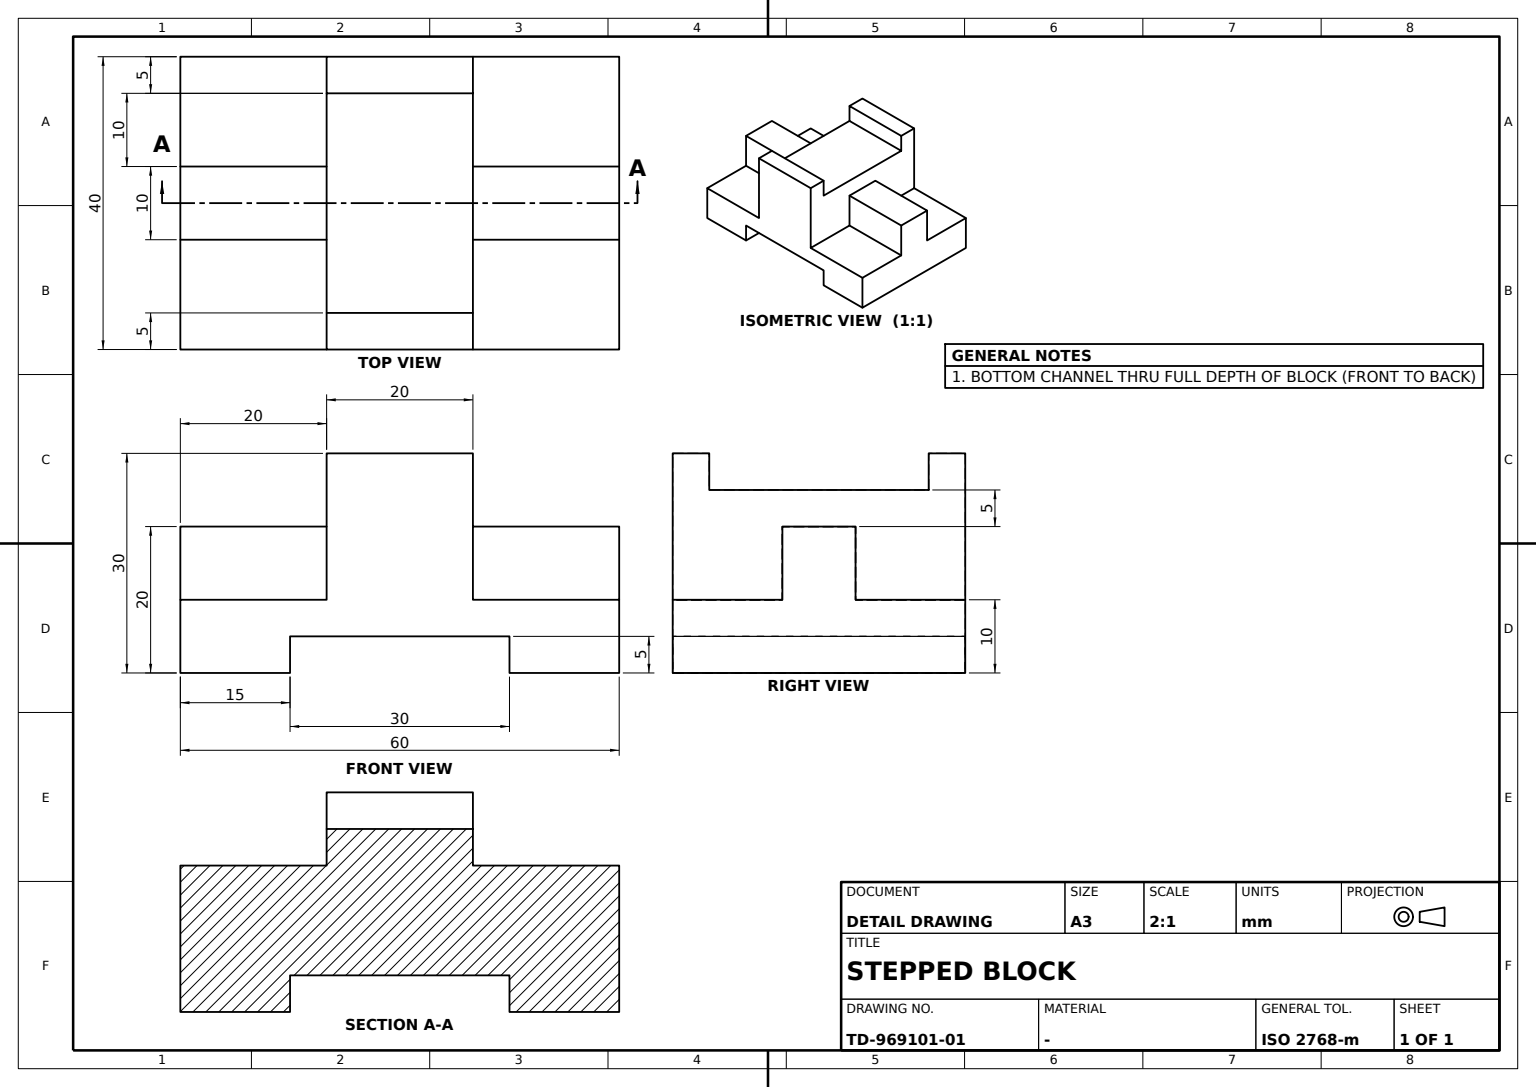
ISO-10303-21;
HEADER;
FILE_DESCRIPTION((''),'2;1');
FILE_NAME('','',(''),(''),'','','');
FILE_SCHEMA(('AUTOMOTIVE_DESIGN'));
ENDSEC;
DATA;
#1=APPLICATION_CONTEXT('');
#2=PRODUCT_CONTEXT('',#1,'mechanical');
#3=PRODUCT('','','',(#2));
#4=PRODUCT_DEFINITION_FORMATION('','',#3);
#5=PRODUCT_DEFINITION_CONTEXT('',#1,'design');
#6=PRODUCT_DEFINITION('','',#4,#5);
#7=PRODUCT_DEFINITION_SHAPE('','',#6);
#8=(LENGTH_UNIT()NAMED_UNIT(*)SI_UNIT(.MILLI.,.METRE.));
#9=(NAMED_UNIT(*)PLANE_ANGLE_UNIT()SI_UNIT($,.RADIAN.));
#10=(NAMED_UNIT(*)SI_UNIT($,.STERADIAN.)SOLID_ANGLE_UNIT());
#11=UNCERTAINTY_MEASURE_WITH_UNIT(LENGTH_MEASURE(0.005),#8,'distance_accuracy_value','');
#12=(GEOMETRIC_REPRESENTATION_CONTEXT(3)GLOBAL_UNCERTAINTY_ASSIGNED_CONTEXT((#11))GLOBAL_UNIT_ASSIGNED_CONTEXT((#8,#9,#10))REPRESENTATION_CONTEXT('',''));
#13=CARTESIAN_POINT('',(-10.,-5.,25.));
#14=VERTEX_POINT('',#13);
#15=CARTESIAN_POINT('',(-10.,-35.,25.));
#16=VERTEX_POINT('',#15);
#17=DIRECTION('',(0.,-1.,0.));
#18=VECTOR('',#17,1000.);
#19=LINE('',#13,#18);
#20=EDGE_CURVE('',#14,#16,#19,.T.);
#21=ORIENTED_EDGE('',*,*,#20,.T.);
#22=CARTESIAN_POINT('',(10.,-35.,25.));
#23=VERTEX_POINT('',#22);
#24=CARTESIAN_POINT('',(0.,-35.,25.));
#25=DIRECTION('',(-1.,0.,0.));
#26=VECTOR('',#25,1000.);
#27=LINE('',#24,#26);
#28=EDGE_CURVE('',#23,#16,#27,.T.);
#29=ORIENTED_EDGE('',*,*,#28,.F.);
#30=CARTESIAN_POINT('',(10.,-5.,25.));
#31=VERTEX_POINT('',#30);
#32=CARTESIAN_POINT('',(10.,0.,25.));
#33=LINE('',#32,#18);
#34=EDGE_CURVE('',#31,#23,#33,.T.);
#35=ORIENTED_EDGE('',*,*,#34,.F.);
#36=CARTESIAN_POINT('',(0.,-5.,25.));
#37=LINE('',#36,#26);
#38=EDGE_CURVE('',#31,#14,#37,.T.);
#39=ORIENTED_EDGE('',*,*,#38,.T.);
#40=EDGE_LOOP('',(#21,#29,#35,#39));
#41=FACE_BOUND('',#40,.T.);
#42=DIRECTION('',(0.,0.,-1.));
#43=AXIS2_PLACEMENT_3D('',#36,#42,#17);
#44=PLANE('',#43);
#45=ADVANCED_FACE('',(#41),#44,.F.);
#46=CARTESIAN_POINT('',(-10.,-25.,10.));
#47=VERTEX_POINT('',#46);
#48=CARTESIAN_POINT('',(-10.,-40.,10.));
#49=VERTEX_POINT('',#48);
#50=CARTESIAN_POINT('',(-10.,0.,10.));
#51=LINE('',#50,#18);
#52=EDGE_CURVE('',#47,#49,#51,.T.);
#53=ORIENTED_EDGE('',*,*,#52,.F.);
#54=CARTESIAN_POINT('',(-30.,-25.,10.));
#55=VERTEX_POINT('',#54);
#56=CARTESIAN_POINT('',(0.,-25.,10.));
#57=DIRECTION('',(1.,0.,0.));
#58=VECTOR('',#57,1000.);
#59=LINE('',#56,#58);
#60=EDGE_CURVE('',#55,#47,#59,.T.);
#61=ORIENTED_EDGE('',*,*,#60,.F.);
#62=CARTESIAN_POINT('',(-30.,-40.,10.));
#63=VERTEX_POINT('',#62);
#64=CARTESIAN_POINT('',(-30.,0.,10.));
#65=LINE('',#64,#18);
#66=EDGE_CURVE('',#55,#63,#65,.T.);
#67=ORIENTED_EDGE('',*,*,#66,.T.);
#68=LINE('',#62,#58);
#69=EDGE_CURVE('',#63,#49,#68,.T.);
#70=ORIENTED_EDGE('',*,*,#69,.T.);
#71=EDGE_LOOP('',(#53,#61,#67,#70));
#72=FACE_BOUND('',#71,.T.);
#73=AXIS2_PLACEMENT_3D('',#64,#42,#57);
#74=PLANE('',#73);
#75=ADVANCED_FACE('',(#72),#74,.F.);
#76=CARTESIAN_POINT('',(-10.,-25.,20.));
#77=VERTEX_POINT('',#76);
#78=DIRECTION('',(0.,0.,1.));
#79=VECTOR('',#78,1000.);
#80=LINE('',#76,#79);
#81=EDGE_CURVE('',#47,#77,#80,.T.);
#82=ORIENTED_EDGE('',*,*,#81,.T.);
#83=CARTESIAN_POINT('',(-30.,-25.,20.));
#84=VERTEX_POINT('',#83);
#85=CARTESIAN_POINT('',(0.,-25.,20.));
#86=LINE('',#85,#58);
#87=EDGE_CURVE('',#84,#77,#86,.T.);
#88=ORIENTED_EDGE('',*,*,#87,.F.);
#89=CARTESIAN_POINT('',(-30.,-25.,0.));
#90=VECTOR('',#42,1000.);
#91=LINE('',#89,#90);
#92=EDGE_CURVE('',#84,#55,#91,.T.);
#93=ORIENTED_EDGE('',*,*,#92,.T.);
#94=ORIENTED_EDGE('',*,*,#60,.T.);
#95=EDGE_LOOP('',(#82,#88,#93,#94));
#96=FACE_BOUND('',#95,.T.);
#97=AXIS2_PLACEMENT_3D('',#85,#17,#42);
#98=PLANE('',#97);
#99=ADVANCED_FACE('',(#96),#98,.T.);
#100=CARTESIAN_POINT('',(10.,-35.,30.));
#101=VERTEX_POINT('',#100);
#102=CARTESIAN_POINT('',(10.,-40.,30.));
#103=VERTEX_POINT('',#102);
#104=CARTESIAN_POINT('',(10.,0.,30.));
#105=LINE('',#104,#18);
#106=EDGE_CURVE('',#101,#103,#105,.T.);
#107=ORIENTED_EDGE('',*,*,#106,.T.);
#108=CARTESIAN_POINT('',(10.,-40.,10.));
#109=VERTEX_POINT('',#108);
#110=LINE('',#102,#90);
#111=EDGE_CURVE('',#103,#109,#110,.T.);
#112=ORIENTED_EDGE('',*,*,#111,.T.);
#113=CARTESIAN_POINT('',(10.,-25.,10.));
#114=VERTEX_POINT('',#113);
#115=CARTESIAN_POINT('',(10.,0.,10.));
#116=LINE('',#115,#18);
#117=EDGE_CURVE('',#114,#109,#116,.T.);
#118=ORIENTED_EDGE('',*,*,#117,.F.);
#119=CARTESIAN_POINT('',(10.,-25.,20.));
#120=VERTEX_POINT('',#119);
#121=CARTESIAN_POINT('',(10.,-25.,30.));
#122=LINE('',#121,#79);
#123=EDGE_CURVE('',#114,#120,#122,.T.);
#124=ORIENTED_EDGE('',*,*,#123,.T.);
#125=CARTESIAN_POINT('',(10.,-15.,20.));
#126=VERTEX_POINT('',#125);
#127=DIRECTION('',(0.,1.,0.));
#128=VECTOR('',#127,1000.);
#129=LINE('',#119,#128);
#130=EDGE_CURVE('',#120,#126,#129,.T.);
#131=ORIENTED_EDGE('',*,*,#130,.T.);
#132=CARTESIAN_POINT('',(10.,-15.,10.));
#133=VERTEX_POINT('',#132);
#134=LINE('',#132,#79);
#135=EDGE_CURVE('',#133,#126,#134,.T.);
#136=ORIENTED_EDGE('',*,*,#135,.F.);
#137=VERTEX_POINT('',#115);
#138=EDGE_CURVE('',#137,#133,#116,.T.);
#139=ORIENTED_EDGE('',*,*,#138,.F.);
#140=VERTEX_POINT('',#104);
#141=LINE('',#104,#90);
#142=EDGE_CURVE('',#140,#137,#141,.T.);
#143=ORIENTED_EDGE('',*,*,#142,.F.);
#144=CARTESIAN_POINT('',(10.,-5.,30.));
#145=VERTEX_POINT('',#144);
#146=EDGE_CURVE('',#140,#145,#105,.T.);
#147=ORIENTED_EDGE('',*,*,#146,.T.);
#148=LINE('',#144,#79);
#149=EDGE_CURVE('',#31,#145,#148,.T.);
#150=ORIENTED_EDGE('',*,*,#149,.F.);
#151=ORIENTED_EDGE('',*,*,#34,.T.);
#152=LINE('',#100,#90);
#153=EDGE_CURVE('',#101,#23,#152,.T.);
#154=ORIENTED_EDGE('',*,*,#153,.F.);
#155=EDGE_LOOP('',(#107,#112,#118,#124,#131,#136,#139,#143,#147,#150,#151,#154));
#156=FACE_BOUND('',#155,.T.);
#157=AXIS2_PLACEMENT_3D('',#104,#25,#42);
#158=PLANE('',#157);
#159=ADVANCED_FACE('',(#156),#158,.F.);
#160=CARTESIAN_POINT('',(-30.,-15.,10.));
#161=VERTEX_POINT('',#160);
#162=CARTESIAN_POINT('',(-10.,-15.,10.));
#163=VERTEX_POINT('',#162);
#164=LINE('',#160,#58);
#165=EDGE_CURVE('',#161,#163,#164,.T.);
#166=ORIENTED_EDGE('',*,*,#165,.F.);
#167=CARTESIAN_POINT('',(-30.,-15.,20.));
#168=VERTEX_POINT('',#167);
#169=CARTESIAN_POINT('',(-30.,-15.,0.));
#170=LINE('',#169,#79);
#171=EDGE_CURVE('',#161,#168,#170,.T.);
#172=ORIENTED_EDGE('',*,*,#171,.T.);
#173=CARTESIAN_POINT('',(-10.,-15.,20.));
#174=VERTEX_POINT('',#173);
#175=CARTESIAN_POINT('',(0.,-15.,20.));
#176=LINE('',#175,#58);
#177=EDGE_CURVE('',#168,#174,#176,.T.);
#178=ORIENTED_EDGE('',*,*,#177,.T.);
#179=LINE('',#162,#79);
#180=EDGE_CURVE('',#163,#174,#179,.T.);
#181=ORIENTED_EDGE('',*,*,#180,.F.);
#182=EDGE_LOOP('',(#166,#172,#178,#181));
#183=FACE_BOUND('',#182,.T.);
#184=CARTESIAN_POINT('',(0.,-15.,10.));
#185=AXIS2_PLACEMENT_3D('',#184,#127,#78);
#186=PLANE('',#185);
#187=ADVANCED_FACE('',(#183),#186,.T.);
#188=CARTESIAN_POINT('',(30.,0.,10.));
#189=VERTEX_POINT('',#188);
#190=LINE('',#64,#58);
#191=EDGE_CURVE('',#137,#189,#190,.T.);
#192=ORIENTED_EDGE('',*,*,#191,.F.);
#193=ORIENTED_EDGE('',*,*,#138,.T.);
#194=CARTESIAN_POINT('',(30.,-15.,10.));
#195=VERTEX_POINT('',#194);
#196=EDGE_CURVE('',#133,#195,#164,.T.);
#197=ORIENTED_EDGE('',*,*,#196,.T.);
#198=LINE('',#188,#18);
#199=EDGE_CURVE('',#189,#195,#198,.T.);
#200=ORIENTED_EDGE('',*,*,#199,.F.);
#201=EDGE_LOOP('',(#192,#193,#197,#200));
#202=FACE_BOUND('',#201,.T.);
#203=ADVANCED_FACE('',(#202),#74,.F.);
#204=VERTEX_POINT('',#50);
#205=EDGE_CURVE('',#204,#163,#51,.T.);
#206=ORIENTED_EDGE('',*,*,#205,.T.);
#207=ORIENTED_EDGE('',*,*,#180,.T.);
#208=CARTESIAN_POINT('',(-10.,0.,20.));
#209=LINE('',#208,#128);
#210=EDGE_CURVE('',#77,#174,#209,.T.);
#211=ORIENTED_EDGE('',*,*,#210,.F.);
#212=ORIENTED_EDGE('',*,*,#81,.F.);
#213=ORIENTED_EDGE('',*,*,#52,.T.);
#214=CARTESIAN_POINT('',(-10.,-40.,30.));
#215=VERTEX_POINT('',#214);
#216=LINE('',#48,#79);
#217=EDGE_CURVE('',#49,#215,#216,.T.);
#218=ORIENTED_EDGE('',*,*,#217,.T.);
#219=CARTESIAN_POINT('',(-10.,-35.,30.));
#220=VERTEX_POINT('',#219);
#221=CARTESIAN_POINT('',(-10.,0.,30.));
#222=LINE('',#221,#18);
#223=EDGE_CURVE('',#220,#215,#222,.T.);
#224=ORIENTED_EDGE('',*,*,#223,.F.);
#225=LINE('',#219,#90);
#226=EDGE_CURVE('',#220,#16,#225,.T.);
#227=ORIENTED_EDGE('',*,*,#226,.T.);
#228=ORIENTED_EDGE('',*,*,#20,.F.);
#229=CARTESIAN_POINT('',(-10.,-5.,30.));
#230=VERTEX_POINT('',#229);
#231=LINE('',#13,#79);
#232=EDGE_CURVE('',#14,#230,#231,.T.);
#233=ORIENTED_EDGE('',*,*,#232,.T.);
#234=VERTEX_POINT('',#221);
#235=EDGE_CURVE('',#234,#230,#222,.T.);
#236=ORIENTED_EDGE('',*,*,#235,.F.);
#237=LINE('',#50,#79);
#238=EDGE_CURVE('',#204,#234,#237,.T.);
#239=ORIENTED_EDGE('',*,*,#238,.F.);
#240=EDGE_LOOP('',(#206,#207,#211,#212,#213,#218,#224,#227,#228,#233,#236,#239));
#241=FACE_BOUND('',#240,.T.);
#242=AXIS2_PLACEMENT_3D('',#50,#57,#78);
#243=PLANE('',#242);
#244=ADVANCED_FACE('',(#241),#243,.F.);
#245=CARTESIAN_POINT('',(30.,-25.,20.));
#246=VERTEX_POINT('',#245);
#247=CARTESIAN_POINT('',(30.,-25.,10.));
#248=VERTEX_POINT('',#247);
#249=LINE('',#245,#90);
#250=EDGE_CURVE('',#246,#248,#249,.T.);
#251=ORIENTED_EDGE('',*,*,#250,.F.);
#252=EDGE_CURVE('',#120,#246,#86,.T.);
#253=ORIENTED_EDGE('',*,*,#252,.F.);
#254=ORIENTED_EDGE('',*,*,#123,.F.);
#255=EDGE_CURVE('',#114,#248,#59,.T.);
#256=ORIENTED_EDGE('',*,*,#255,.T.);
#257=EDGE_LOOP('',(#251,#253,#254,#256));
#258=FACE_BOUND('',#257,.T.);
#259=ADVANCED_FACE('',(#258),#98,.T.);
#260=LINE('',#221,#58);
#261=EDGE_CURVE('',#234,#140,#260,.T.);
#262=ORIENTED_EDGE('',*,*,#261,.F.);
#263=ORIENTED_EDGE('',*,*,#235,.T.);
#264=LINE('',#229,#26);
#265=EDGE_CURVE('',#145,#230,#264,.T.);
#266=ORIENTED_EDGE('',*,*,#265,.F.);
#267=ORIENTED_EDGE('',*,*,#146,.F.);
#268=EDGE_LOOP('',(#262,#263,#266,#267));
#269=FACE_BOUND('',#268,.T.);
#270=AXIS2_PLACEMENT_3D('',#221,#42,#57);
#271=PLANE('',#270);
#272=ADVANCED_FACE('',(#269),#271,.F.);
#273=ORIENTED_EDGE('',*,*,#117,.T.);
#274=CARTESIAN_POINT('',(30.,-40.,10.));
#275=VERTEX_POINT('',#274);
#276=EDGE_CURVE('',#109,#275,#68,.T.);
#277=ORIENTED_EDGE('',*,*,#276,.T.);
#278=EDGE_CURVE('',#248,#275,#198,.T.);
#279=ORIENTED_EDGE('',*,*,#278,.F.);
#280=ORIENTED_EDGE('',*,*,#255,.F.);
#281=EDGE_LOOP('',(#273,#277,#279,#280));
#282=FACE_BOUND('',#281,.T.);
#283=ADVANCED_FACE('',(#282),#74,.F.);
#284=CARTESIAN_POINT('',(30.,-40.,0.));
#285=VERTEX_POINT('',#284);
#286=CARTESIAN_POINT('',(15.,-40.,0.));
#287=VERTEX_POINT('',#286);
#288=LINE('',#284,#26);
#289=EDGE_CURVE('',#285,#287,#288,.T.);
#290=ORIENTED_EDGE('',*,*,#289,.T.);
#291=CARTESIAN_POINT('',(15.,0.,0.));
#292=VERTEX_POINT('',#291);
#293=LINE('',#291,#18);
#294=EDGE_CURVE('',#292,#287,#293,.T.);
#295=ORIENTED_EDGE('',*,*,#294,.F.);
#296=CARTESIAN_POINT('',(30.,0.,0.));
#297=VERTEX_POINT('',#296);
#298=LINE('',#296,#26);
#299=EDGE_CURVE('',#297,#292,#298,.T.);
#300=ORIENTED_EDGE('',*,*,#299,.F.);
#301=LINE('',#296,#18);
#302=EDGE_CURVE('',#297,#285,#301,.T.);
#303=ORIENTED_EDGE('',*,*,#302,.T.);
#304=EDGE_LOOP('',(#290,#295,#300,#303));
#305=FACE_BOUND('',#304,.T.);
#306=AXIS2_PLACEMENT_3D('',#296,#78,#25);
#307=PLANE('',#306);
#308=ADVANCED_FACE('',(#305),#307,.F.);
#309=ORIENTED_EDGE('',*,*,#106,.F.);
#310=CARTESIAN_POINT('',(0.,-35.,30.));
#311=LINE('',#310,#26);
#312=EDGE_CURVE('',#101,#220,#311,.T.);
#313=ORIENTED_EDGE('',*,*,#312,.T.);
#314=ORIENTED_EDGE('',*,*,#223,.T.);
#315=LINE('',#214,#58);
#316=EDGE_CURVE('',#215,#103,#315,.T.);
#317=ORIENTED_EDGE('',*,*,#316,.T.);
#318=EDGE_LOOP('',(#309,#313,#314,#317));
#319=FACE_BOUND('',#318,.T.);
#320=ADVANCED_FACE('',(#319),#271,.F.);
#321=CARTESIAN_POINT('',(-15.,0.,5.));
#322=VERTEX_POINT('',#321);
#323=CARTESIAN_POINT('',(-15.,-40.,5.));
#324=VERTEX_POINT('',#323);
#325=LINE('',#321,#18);
#326=EDGE_CURVE('',#322,#324,#325,.T.);
#327=ORIENTED_EDGE('',*,*,#326,.T.);
#328=CARTESIAN_POINT('',(-15.,-40.,0.));
#329=VERTEX_POINT('',#328);
#330=LINE('',#323,#90);
#331=EDGE_CURVE('',#324,#329,#330,.T.);
#332=ORIENTED_EDGE('',*,*,#331,.T.);
#333=CARTESIAN_POINT('',(-15.,0.,0.));
#334=VERTEX_POINT('',#333);
#335=LINE('',#333,#18);
#336=EDGE_CURVE('',#334,#329,#335,.T.);
#337=ORIENTED_EDGE('',*,*,#336,.F.);
#338=LINE('',#321,#90);
#339=EDGE_CURVE('',#322,#334,#338,.T.);
#340=ORIENTED_EDGE('',*,*,#339,.F.);
#341=EDGE_LOOP('',(#327,#332,#337,#340));
#342=FACE_BOUND('',#341,.T.);
#343=AXIS2_PLACEMENT_3D('',#321,#25,#42);
#344=PLANE('',#343);
#345=ADVANCED_FACE('',(#342),#344,.F.);
#346=ORIENTED_EDGE('',*,*,#92,.F.);
#347=CARTESIAN_POINT('',(-30.,0.,20.));
#348=LINE('',#347,#128);
#349=EDGE_CURVE('',#84,#168,#348,.T.);
#350=ORIENTED_EDGE('',*,*,#349,.T.);
#351=ORIENTED_EDGE('',*,*,#171,.F.);
#352=VERTEX_POINT('',#64);
#353=EDGE_CURVE('',#352,#161,#65,.T.);
#354=ORIENTED_EDGE('',*,*,#353,.F.);
#355=CARTESIAN_POINT('',(-30.,0.,0.));
#356=VERTEX_POINT('',#355);
#357=LINE('',#355,#79);
#358=EDGE_CURVE('',#356,#352,#357,.T.);
#359=ORIENTED_EDGE('',*,*,#358,.F.);
#360=CARTESIAN_POINT('',(-30.,-40.,0.));
#361=VERTEX_POINT('',#360);
#362=LINE('',#355,#18);
#363=EDGE_CURVE('',#356,#361,#362,.T.);
#364=ORIENTED_EDGE('',*,*,#363,.T.);
#365=LINE('',#360,#79);
#366=EDGE_CURVE('',#361,#63,#365,.T.);
#367=ORIENTED_EDGE('',*,*,#366,.T.);
#368=ORIENTED_EDGE('',*,*,#66,.F.);
#369=EDGE_LOOP('',(#346,#350,#351,#354,#359,#364,#367,#368));
#370=FACE_BOUND('',#369,.T.);
#371=AXIS2_PLACEMENT_3D('',#355,#57,#78);
#372=PLANE('',#371);
#373=ADVANCED_FACE('',(#370),#372,.F.);
#374=CARTESIAN_POINT('',(15.,-40.,5.));
#375=VERTEX_POINT('',#374);
#376=LINE('',#374,#26);
#377=EDGE_CURVE('',#375,#324,#376,.T.);
#378=ORIENTED_EDGE('',*,*,#377,.T.);
#379=ORIENTED_EDGE('',*,*,#326,.F.);
#380=CARTESIAN_POINT('',(15.,0.,5.));
#381=VERTEX_POINT('',#380);
#382=LINE('',#380,#26);
#383=EDGE_CURVE('',#381,#322,#382,.T.);
#384=ORIENTED_EDGE('',*,*,#383,.F.);
#385=LINE('',#380,#18);
#386=EDGE_CURVE('',#381,#375,#385,.T.);
#387=ORIENTED_EDGE('',*,*,#386,.T.);
#388=EDGE_LOOP('',(#378,#379,#384,#387));
#389=FACE_BOUND('',#388,.T.);
#390=AXIS2_PLACEMENT_3D('',#380,#78,#25);
#391=PLANE('',#390);
#392=ADVANCED_FACE('',(#389),#391,.F.);
#393=ORIENTED_EDGE('',*,*,#261,.T.);
#394=ORIENTED_EDGE('',*,*,#142,.T.);
#395=ORIENTED_EDGE('',*,*,#191,.T.);
#396=LINE('',#188,#90);
#397=EDGE_CURVE('',#189,#297,#396,.T.);
#398=ORIENTED_EDGE('',*,*,#397,.T.);
#399=ORIENTED_EDGE('',*,*,#299,.T.);
#400=LINE('',#291,#79);
#401=EDGE_CURVE('',#292,#381,#400,.T.);
#402=ORIENTED_EDGE('',*,*,#401,.T.);
#403=ORIENTED_EDGE('',*,*,#383,.T.);
#404=ORIENTED_EDGE('',*,*,#339,.T.);
#405=EDGE_CURVE('',#334,#356,#298,.T.);
#406=ORIENTED_EDGE('',*,*,#405,.T.);
#407=ORIENTED_EDGE('',*,*,#358,.T.);
#408=EDGE_CURVE('',#352,#204,#190,.T.);
#409=ORIENTED_EDGE('',*,*,#408,.T.);
#410=ORIENTED_EDGE('',*,*,#238,.T.);
#411=EDGE_LOOP('',(#393,#394,#395,#398,#399,#402,#403,#404,#406,#407,#409,#410));
#412=FACE_BOUND('',#411,.T.);
#413=CARTESIAN_POINT('',(0.,0.,0.));
#414=AXIS2_PLACEMENT_3D('',#413,#127,#25);
#415=PLANE('',#414);
#416=ADVANCED_FACE('',(#412),#415,.T.);
#417=LINE('',#286,#79);
#418=EDGE_CURVE('',#287,#375,#417,.T.);
#419=ORIENTED_EDGE('',*,*,#418,.F.);
#420=ORIENTED_EDGE('',*,*,#289,.F.);
#421=LINE('',#274,#90);
#422=EDGE_CURVE('',#275,#285,#421,.T.);
#423=ORIENTED_EDGE('',*,*,#422,.F.);
#424=ORIENTED_EDGE('',*,*,#276,.F.);
#425=ORIENTED_EDGE('',*,*,#111,.F.);
#426=ORIENTED_EDGE('',*,*,#316,.F.);
#427=ORIENTED_EDGE('',*,*,#217,.F.);
#428=ORIENTED_EDGE('',*,*,#69,.F.);
#429=ORIENTED_EDGE('',*,*,#366,.F.);
#430=EDGE_CURVE('',#329,#361,#288,.T.);
#431=ORIENTED_EDGE('',*,*,#430,.F.);
#432=ORIENTED_EDGE('',*,*,#331,.F.);
#433=ORIENTED_EDGE('',*,*,#377,.F.);
#434=EDGE_LOOP('',(#419,#420,#423,#424,#425,#426,#427,#428,#429,#431,#432,#433));
#435=FACE_BOUND('',#434,.T.);
#436=CARTESIAN_POINT('',(0.,-40.,0.));
#437=AXIS2_PLACEMENT_3D('',#436,#127,#25);
#438=PLANE('',#437);
#439=ADVANCED_FACE('',(#435),#438,.F.);
#440=ORIENTED_EDGE('',*,*,#252,.T.);
#441=CARTESIAN_POINT('',(30.,-15.,20.));
#442=VERTEX_POINT('',#441);
#443=LINE('',#245,#128);
#444=EDGE_CURVE('',#246,#442,#443,.T.);
#445=ORIENTED_EDGE('',*,*,#444,.T.);
#446=EDGE_CURVE('',#126,#442,#176,.T.);
#447=ORIENTED_EDGE('',*,*,#446,.F.);
#448=ORIENTED_EDGE('',*,*,#130,.F.);
#449=EDGE_LOOP('',(#440,#445,#447,#448));
#450=FACE_BOUND('',#449,.T.);
#451=AXIS2_PLACEMENT_3D('',#85,#42,#127);
#452=PLANE('',#451);
#453=ADVANCED_FACE('',(#450),#452,.F.);
#454=ORIENTED_EDGE('',*,*,#278,.T.);
#455=ORIENTED_EDGE('',*,*,#422,.T.);
#456=ORIENTED_EDGE('',*,*,#302,.F.);
#457=ORIENTED_EDGE('',*,*,#397,.F.);
#458=ORIENTED_EDGE('',*,*,#199,.T.);
#459=LINE('',#194,#79);
#460=EDGE_CURVE('',#195,#442,#459,.T.);
#461=ORIENTED_EDGE('',*,*,#460,.T.);
#462=ORIENTED_EDGE('',*,*,#444,.F.);
#463=ORIENTED_EDGE('',*,*,#250,.T.);
#464=EDGE_LOOP('',(#454,#455,#456,#457,#458,#461,#462,#463));
#465=FACE_BOUND('',#464,.T.);
#466=AXIS2_PLACEMENT_3D('',#188,#25,#42);
#467=PLANE('',#466);
#468=ADVANCED_FACE('',(#465),#467,.F.);
#469=ORIENTED_EDGE('',*,*,#153,.T.);
#470=ORIENTED_EDGE('',*,*,#28,.T.);
#471=ORIENTED_EDGE('',*,*,#226,.F.);
#472=ORIENTED_EDGE('',*,*,#312,.F.);
#473=EDGE_LOOP('',(#469,#470,#471,#472));
#474=FACE_BOUND('',#473,.T.);
#475=AXIS2_PLACEMENT_3D('',#310,#127,#42);
#476=PLANE('',#475);
#477=ADVANCED_FACE('',(#474),#476,.T.);
#478=ORIENTED_EDGE('',*,*,#232,.F.);
#479=ORIENTED_EDGE('',*,*,#38,.F.);
#480=ORIENTED_EDGE('',*,*,#149,.T.);
#481=ORIENTED_EDGE('',*,*,#265,.T.);
#482=EDGE_LOOP('',(#478,#479,#480,#481));
#483=FACE_BOUND('',#482,.T.);
#484=AXIS2_PLACEMENT_3D('',#36,#17,#78);
#485=PLANE('',#484);
#486=ADVANCED_FACE('',(#483),#485,.T.);
#487=ORIENTED_EDGE('',*,*,#363,.F.);
#488=ORIENTED_EDGE('',*,*,#405,.F.);
#489=ORIENTED_EDGE('',*,*,#336,.T.);
#490=ORIENTED_EDGE('',*,*,#430,.T.);
#491=EDGE_LOOP('',(#487,#488,#489,#490));
#492=FACE_BOUND('',#491,.T.);
#493=ADVANCED_FACE('',(#492),#307,.F.);
#494=ORIENTED_EDGE('',*,*,#165,.T.);
#495=ORIENTED_EDGE('',*,*,#205,.F.);
#496=ORIENTED_EDGE('',*,*,#408,.F.);
#497=ORIENTED_EDGE('',*,*,#353,.T.);
#498=EDGE_LOOP('',(#494,#495,#496,#497));
#499=FACE_BOUND('',#498,.T.);
#500=ADVANCED_FACE('',(#499),#74,.F.);
#501=ORIENTED_EDGE('',*,*,#210,.T.);
#502=ORIENTED_EDGE('',*,*,#177,.F.);
#503=ORIENTED_EDGE('',*,*,#349,.F.);
#504=ORIENTED_EDGE('',*,*,#87,.T.);
#505=EDGE_LOOP('',(#501,#502,#503,#504));
#506=FACE_BOUND('',#505,.T.);
#507=ADVANCED_FACE('',(#506),#452,.F.);
#508=ORIENTED_EDGE('',*,*,#418,.T.);
#509=ORIENTED_EDGE('',*,*,#386,.F.);
#510=ORIENTED_EDGE('',*,*,#401,.F.);
#511=ORIENTED_EDGE('',*,*,#294,.T.);
#512=EDGE_LOOP('',(#508,#509,#510,#511));
#513=FACE_BOUND('',#512,.T.);
#514=AXIS2_PLACEMENT_3D('',#291,#57,#78);
#515=PLANE('',#514);
#516=ADVANCED_FACE('',(#513),#515,.F.);
#517=ORIENTED_EDGE('',*,*,#135,.T.);
#518=ORIENTED_EDGE('',*,*,#446,.T.);
#519=ORIENTED_EDGE('',*,*,#460,.F.);
#520=ORIENTED_EDGE('',*,*,#196,.F.);
#521=EDGE_LOOP('',(#517,#518,#519,#520));
#522=FACE_BOUND('',#521,.T.);
#523=ADVANCED_FACE('',(#522),#186,.T.);
#524=CLOSED_SHELL('',(#45,#75,#99,#159,#187,#203,#244,#259,#272,#283,#308,#320,#345,#373,#392,#416,#439,#453,#468,#477,#486,#493,#500,#507,#516,#523));
#525=MANIFOLD_SOLID_BREP('',#524);
#526=ADVANCED_BREP_SHAPE_REPRESENTATION('',(#525),#12);
#527=SHAPE_DEFINITION_REPRESENTATION(#7,#526);
ENDSEC;
END-ISO-10303-21;
